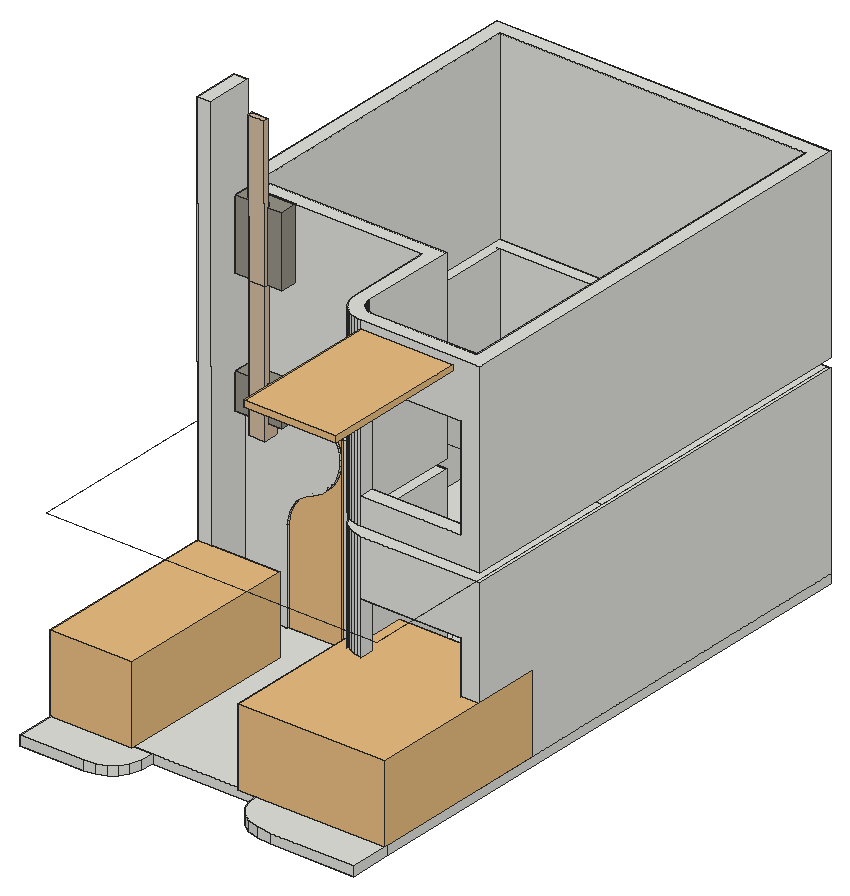
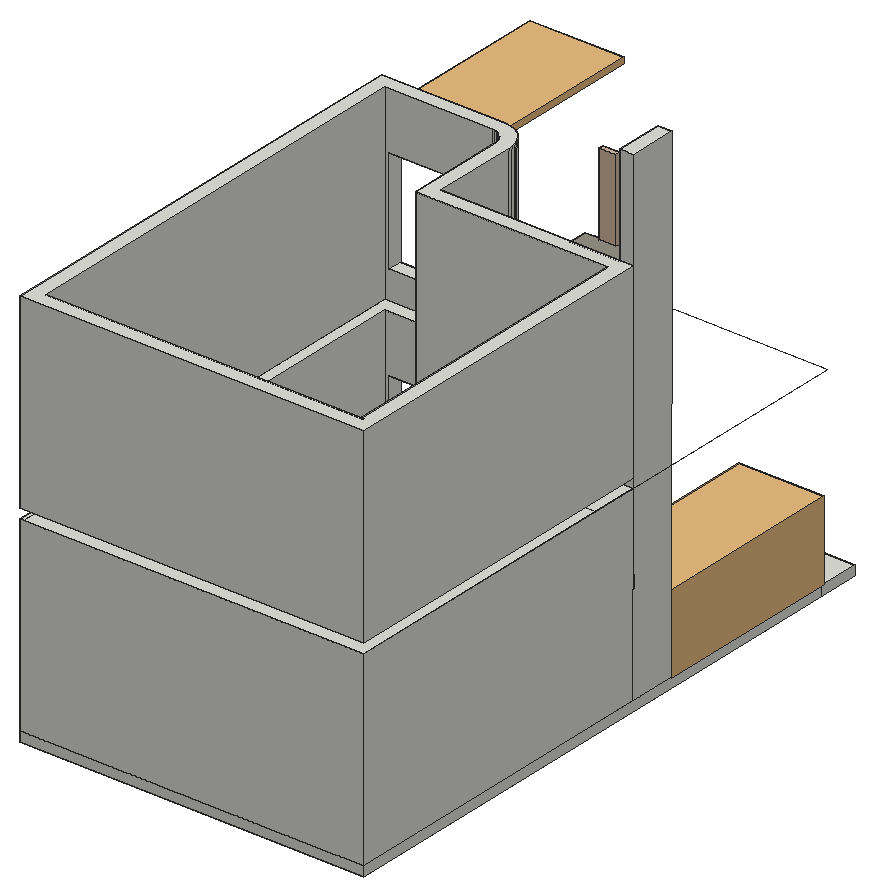
# SketchUp Ruby script. Lengths in inches.
U = 1.inch
M = Sketchup.active_model
def pt(a) = Geom::Point3d.new(a.map { |v| v * U })
def face(e, loops, mat)
  f = e.add_face(loops[0].map { |a| pt(a) })
  loops[1..].each { |l| e.add_face(l.map { |a| pt(a) }).erase! }
  f.material = f.back_material = mat if mat
  f
end
# faces: each face lists its corners as indices into pts; further lists are holes
def faces(e, pts, list, mat = nil) = list.each { |f| face(e, (f[0].is_a?(Array) ? f : [f]).map { |l| l.map { |i| pts[i] } }, mat) }
# xy, xz, yz: faces in a plane at the given z, y or x. An outline is a flat list of corners, or four numbers for a rectangle; further outlines are holes
def ring(l) = l.size == 4 ? [[l[0], l[1]], [l[2], l[1]], [l[2], l[3]], [l[0], l[3]]] : l.each_slice(2).to_a
def flat(e, list, mat, &to3) = list.each { |f| face(e, (f[0].is_a?(Array) ? f : [f]).map { |l| ring(l).map { |u, v| to3.(u, v) } }, mat) }
def xy(e, z, list, mat = nil) = flat(e, list, mat) { |x, y| [x, y, z] }
def xz(e, y, list, mat = nil) = flat(e, list, mat) { |x, z| [x, y, z] }
def yz(e, x, list, mat = nil) = flat(e, list, mat) { |y, z| [x, y, z] }
def lines(e, pts, list) = list.each { |a, b| e.add_line(pt(pts[a]), pt(pts[b])) }
# prism: a flat outline (further loops are holes) pulled along v
def prism(e, loops, v, mat = nil)
  f = face(e, loops, mat); d = Geom::Vector3d.new(v.map { |x| x * U })
  f.pushpull(f.normal.samedirection?(d) ? d.length : -d.length)
end
def box(e, o, s, mat = nil) = prism(e, [[o, [o[0] + s[0], o[1], o[2]], [o[0] + s[0], o[1] + s[1], o[2]], [o[0], o[1] + s[1], o[2]]]], [0, 0, s[2]], mat)
def at(x, y, z, deg = 0) = Geom::Transformation.translation(pt([x, y, z])) * Geom::Transformation.rotation(ORIGIN, Z_AXIS, deg.degrees)
def axes(o, x, y, z) = Geom::Transformation.new([*x, 0, *y, 0, *z, 0, *pt(o).to_a, 1])
def part(name) = M.definitions.add(name)
# library, detail: a bought-in or finely detailed component or shape, given as its bounding box
def library(name, o, s) = part(name).tap { |d| box(d.entities, o, s) }
def detail(e, o, s) = box(e.add_group.entities, o, s)
def put(e, d, t, mat = nil) = e.add_instance(d, t).tap { |i| i.material = mat if mat }
def group(e, t, mat = nil) = e.add_group.tap { |g| g.transformation = t; g.material = mat if mat }.entities
root = M.entities
M.materials.add("[Formica Graystone]").color = [149, 146, 135]
M.materials.add("[Formica Laminate Light]").color = [213, 189, 164]
M.materials.add("[Wood Cherry Original]").color = [152, 86, 42]
c1 = part("Group316\#3")
p = [[0,0,0],[0,0,-89.7],[-16.49,0,-89.7],[107.35,-183.05,0],[-107.35,-183.05,0],[107.35,183.05,0],
  [107.35,0,0],[-107.35,183.05,0],[16.49,0,-89.7],[-107.35,0,0],[0,0,-145.2]]
lines(c1.entities,p,[[0,1],[1,2],[3,4],[5,6],[7,5],[1,8],[9,0],[0,6],[8,10],[4,9],[6,3],[2,10],
  [9,7]])
c2 = part("Rectangle Light")
put(c2.entities,c1,at(0,0,0))
c3 = part("Group\#13")
prism(c3.entities,[[[0,0,0],[0,27,0],[84,27,0],[83.17,18.75,0],[80.68,12,0],[76.53,6.75,0],[70.71,3,0],[63.24,0.75,0],[54.1,0,0]]],[0,0,6])
c4 = library("Group\#11",[-9.29,0,0],[59.29,4,95])
c5 = library("Group\#10",[-0.5,-0.5,0],[35.9375,1,120.38])
c6 = library("Group123\#1",[-245.88,56.46,51.12],[36,6.2,84])
c7 = library("Group297\#3",[-33.91,-76.98,0],[95.34,119.86,50])
c8 = library("Group297\#2",[-33.91,-76.98,0],[95.34,119.86,50])
xy(root,48,[[132.2,27,195.57,32]])
xz(root,32,[[123.2,0,211.73,48]])
put(root,c2,axes([107.57,204.35,119.99],[1,0,0],[0,-1,0],[0,0,1]))
put(root,c3,axes([217.23,0,-6],[-1,0,0],[0,1,0],[0,0,1]))
g1 = group(root,at(29.625,105.98,-6))
xy(g1,0,[[-29.41,-78.98,-29.41,281.41,187.6,281.41,187.6,-78.98,178.93,-78.98,178.93,-75.77,174.22,-75.77,174.22,-78.98],[174.22,-78.98,174.22,-75.77,178.93,-75.77,178.93,-77.125,178.43,-77.82,177.68,-78.36,176.39,-78.79],[174.22,-78.98,176.39,-78.79,177.68,-78.36,178.43,-77.82,178.93,-77.125,178.93,-78.98]])
xy(g1,6,[[-29.41,-78.98,187.6,281.41]])
xz(g1,-78.98,[[-29.41,0,187.6,6]])
xz(g1,281.41,[[-29.41,0,187.6,6]])
yz(g1,-29.41,[[-78.98,0,281.41,6]])
yz(g1,187.6,[[-78.98,0,281.41,6]])
put(root,c3,axes([0.22,0,-6],[0.77,0,0],[0,1,0],[0,0,1]))
g2 = group(root,at(33.625,101.98,126))
xy(g2,0,[[106.8125,0,104.36,0.16,101.94,0.64,99.61,1.43,97.41,2.52,95.36,3.89,93.51,5.51,91.89,7.36,90.52,9.41,89.43,11.61,88.64,13.94,88.16,16.36,88,18.8125,88,72.51,40,72.51,40,81.51,97,81.51,97,18.8125,97.08,17.53,97.33,16.27,97.75,15.06,98.31,13.91,99.03,12.84,99.875,11.875,100.84,11.03,101.91,10.31,103.06,9.75,104.27,9.33,105.53,9.08,106.8125,9,174.6,9,174.6,276.41,0,276.41,0,285.41,183.6,285.41,183.6,0],[-33.41,72.51,-33.41,285.41,0,285.41,0,276.41,-24.41,276.41,-24.41,81.51,0,81.51,0,72.51],[0,72.51,40,81.51]])
xy(g2,18,[[106.8125,0,171.6,9]])
xy(g2,84,[[106.8125,0,171.6,9]])
xy(g2,120,[[[106.8125,0,183.6,0,183.6,285.41,-33.41,285.41,-33.41,72.51,88,72.51,88,18.8125,88.16,16.36,88.64,13.94,89.43,11.61,90.52,9.41,91.89,7.36,93.51,5.51,95.36,3.89,97.41,2.52,99.61,1.43,101.94,0.64,104.36,0.16],[106.8125,9,105.53,9.08,104.27,9.33,103.06,9.75,101.91,10.31,100.84,11.03,99.875,11.875,99.03,12.84,98.31,13.91,97.75,15.06,97.33,16.27,97.08,17.53,97,18.8125,97,81.51,-24.41,81.51,-24.41,276.41,174.6,276.41,174.6,9]]])
xz(g2,0,[[106.8125,0,183.6,0,183.6,120,106.8125,120,106.8125,84,171.6,84,171.6,18,106.8125,18]])
xz(g2,9,[[106.8125,0,106.8125,18,171.6,18,171.6,84,106.8125,84,106.8125,120,174.6,120,174.6,0]])
xz(g2,72.51,[[-33.41,0,88,120]])
xz(g2,81.51,[[-24.41,0,97,120]])
xz(g2,276.41,[[-26.08,0,-24.41,120],[-24.41,0,174.6,120]])
xz(g2,285.41,[[-33.41,0,183.6,120]])
yz(g2,-33.41,[[42.875,-126.09,41.97,182.5,71.97,182.58,72.51,0,72.875,-126],[72.51,0,285.41,120]])
yz(g2,-24.41,[[42.875,-126.09,72.875,-126,72.51,0,71.97,182.58,41.97,182.5],[81.51,0,276.41,120]])
yz(g2,88,[[18.8125,0,72.51,120]])
yz(g2,97,[[18.8125,0,81.51,120]])
yz(g2,106.8125,[[0,18,9,84]])
yz(g2,171.6,[[0,18,9,84]])
yz(g2,174.6,[[9,0,276.41,120]])
yz(g2,183.6,[[0,0,285.41,120]])
p = [[-24.41,41.97,182.5],[-33.41,41.97,182.5],[-33.41,42.875,-126.09],[-24.41,42.875,-126.09],[-33.41,72.875,-126],[-24.41,72.875,-126],
  [-33.41,72.51,0],[-24.41,72.51,0],[104.36,0.16,0],[106.8125,0,0],[106.8125,0,18],[106.8125,0,84],
  [106.8125,0,120],[104.36,0.16,120],[101.94,0.64,0],[101.94,0.64,120],[99.61,1.43,0],[99.61,1.43,120],
  [97.41,2.52,0],[97.41,2.52,120],[95.36,3.89,0],[95.36,3.89,120],[93.51,5.51,0],[93.51,5.51,120],
  [91.89,7.36,0],[91.89,7.36,120],[90.52,9.41,0],[90.52,9.41,120],[106.8125,9,0],[105.53,9.08,0],
  [105.53,9.08,120],[106.8125,9,120],[106.8125,9,84],[106.8125,9,18],[104.27,9.33,0],[104.27,9.33,120],
  [103.06,9.75,0],[103.06,9.75,120],[89.43,11.61,0],[89.43,11.61,120],[101.91,10.31,0],[101.91,10.31,120],
  [100.84,11.03,0],[100.84,11.03,120],[99.875,11.875,0],[99.875,11.875,120],[88.64,13.94,0],[88.64,13.94,120],
  [99.03,12.84,0],[99.03,12.84,120],[98.31,13.91,0],[98.31,13.91,120],[88.16,16.36,0],[88.16,16.36,120],
  [97.75,15.06,0],[97.75,15.06,120],[97.33,16.27,0],[97.33,16.27,120],[97.08,17.53,0],[97.08,17.53,120],
  [88,18.8125,0],[88,18.8125,120],[97,18.8125,0],[97,18.8125,120],[-33.41,71.97,182.58],[-24.41,71.97,182.58]]
faces(g2,p,[[0,1,2,3],[4,5,3,2],[6,7,5,4],[8,9,10,11,12,13],[14,8,13,15],[16,14,15,17],[18,16,17,19],[20,18,19,21],
  [22,20,21,23],[24,22,23,25],[26,24,25,27],[28,29,30,31,32,33],[29,34,35,30],[34,36,37,35],[38,26,27,39],[36,40,41,37],
  [40,42,43,41],[42,44,45,43],[46,38,39,47],[44,48,49,45],[48,50,51,49],[52,46,47,53],[50,54,55,51],[54,56,57,55],
  [56,58,59,57],[60,52,53,61],[58,62,63,59],[64,65,7,6],[1,0,65,64]])
g3 = group(g2,at(-24.41,72.34,57.67),"[Formica Graystone]")
prism(g3,[[[0,0.18,-63.22],[30.33,0.35,-63.22],[30.39,-10.65,-63.25],[0.0625,-10.81,-63.25]]],[0,-0.07,23.04])
p = [[0.0625,-11.18,62.3],[-0.01,0.82,62.33],[-0.01,0.95,17.01],[0,-0.05,17],[0.0625,-11.05,16.97],[10.46,-10.99,16.97],
  [10.46,-11.125,62.3],[30.39,-11.01,62.3],[20.9375,-11.07,62.3],[20.9375,-10.93,16.97],[30.39,-10.88,16.97],[30.32,1.12,17.01],
  [30.32,0.99,62.33],[0,0.12,-40.18]]
faces(g3,p,[[0,1,2,3,4],[4,5,6,0],[7,8,9,10],[10,9,5,4,3,2,11],[10,11,12,7],[12,11,2,1],[7,12,1,0,6,8]])
lines(g3,p,[[3,13]])
g4 = group(g3,at(10.46,-10.93,16.97),"[Formica Laminate Light]")
p = [[-0.01,0.94,0],[-0.01,1.18,-80.22],[-0.06,11.03,-80.1875],[-0.06,11.0625,-90.1875],[0.01,-1.79,-90.23],[0.01,-2.06,-0.01],
  [10.49,-1.74,-90.23],[10.49,-2,-0.01],[10.42,11.12,-90.1875],[10.42,11.09,-80.1875],[10.48,1.23,-80.22],[10.48,1,0],
  [10.49,-2.28,96.77],[0.01,-2.34,96.77],[-0.01,0.66,96.78],[10.48,0.72,96.78]]
faces(g4,p,[[0,1,2,3,4,5],[5,4,6,7],[7,6,8,9,10,11],[8,6,4,3],[3,2,9,8],[11,10,1,0],[1,10,9,2],[12,13,5,7],
  [13,14,0,5],[15,12,7,11],[5,7,11,0],[14,15,11,0],[14,13,12,15]])
put(g2,c4,axes([116.1,0,111.06],[1,0,0],[0,0,1],[0,-1,0]))
g5 = group(root,at(33.625,101.98,0))
xy(g5,0,[[106.8125,0,104.36,0.16,101.94,0.64,99.61,1.43,97.41,2.52,95.36,3.89,93.51,5.51,91.89,7.36,90.52,9.41,89.43,11.61,88.64,13.94,88.16,16.36,88,18.8125,88,72.51,76,72.51,76,81.51,97,81.51,97,18.8125,97.08,17.53,97.33,16.27,97.75,15.06,98.31,13.91,99.03,12.84,99.875,11.875,100.84,11.03,101.91,10.31,103.06,9.75,104.27,9.33,105.53,9.08,106.8125,9,174.6,9,174.6,276.41,0,276.41,0,285.41,183.6,285.41,183.6,0],[-33.41,69.51,-33.41,285.41,0,285.41,0,276.41,-24.41,276.41,-24.41,81.51,0,81.51,0,69.51],[0,69.51,0,81.51,40,81.51,40,72.51,2.51,72.51,2.51,69.51],[2.51,69.51,3.51,71.01]])
xy(g5,18,[[106.8125,0,171.6,9]])
xy(g5,84,[[106.8125,0,171.6,9],[40,72.51,76,81.51]])
xy(g5,120,[[[106.8125,0,183.6,0,183.6,285.41,-33.41,285.41,-33.41,69.51,33.73,69.51,33.73,72.51,88,72.51,88,18.8125,88.16,16.36,88.64,13.94,89.43,11.61,90.52,9.41,91.89,7.36,93.51,5.51,95.36,3.89,97.41,2.52,99.61,1.43,101.94,0.64,104.36,0.16],[106.8125,9,105.53,9.08,104.27,9.33,103.06,9.75,101.91,10.31,100.84,11.03,99.875,11.875,99.03,12.84,98.31,13.91,97.75,15.06,97.33,16.27,97.08,17.53,97,18.8125,97,81.51,-24.41,81.51,-24.41,276.41,174.6,276.41,174.6,9]]])
xz(g5,0,[[106.8125,0,183.6,0,183.6,120,106.8125,120,106.8125,84,171.6,84,171.6,18,106.8125,18]])
xz(g5,9,[[106.8125,0,106.8125,18,171.6,18,171.6,84,106.8125,84,106.8125,120,174.6,120,174.6,0]])
xz(g5,69.51,[[-33.41,0,3.51,0,3.51,59.97,3.64,62.47,4.01,64.91,4.64,67.3,5.5,69.62,6.6,71.83,7.91,73.92,9.43,75.87,11.14,77.65,13.03,79.25,15.07,80.65,17.24,81.83,19.57,82.81,23,84.33,26.24,86.35,29.16,88.8,31.72,91.63,33.84,94.8,35.51,98.23,36.68,101.86,37.33,105.62,37.44,109.43,37.03,113.22,36.08,116.92,34.66,120.38,33.73,120,-33.41,120]])
xz(g5,72.51,[[2.51,0,40,0,40,84,76,84,76,0,88,0,88,120,33.73,120,35.13,116.6,36.04,113.04,36.44,109.39,36.33,105.72,35.71,102.1,34.58,98.6,32.98,95.3,30.92,92.25,28.47,89.52,25.65,87.16,22.53,85.22,19.17,83.73,16.8,82.74,14.54,81.5,12.42,80.05,10.46,78.38,8.68,76.53,7.09,74.5,5.72,72.32,4.58,70.01,3.68,67.6,3.03,65.11,2.64,62.57,2.51,60]])
xz(g5,81.51,[[-24.41,0,-24.41,120,97,120,97,0,76,0,76,84,40,84,40,0]])
xz(g5,276.41,[[-26.08,0,-24.41,120],[-24.41,0,174.6,120]])
xz(g5,285.41,[[-33.41,0,183.6,120]])
yz(g5,-33.41,[[69.51,0,285.41,120]])
yz(g5,-24.41,[[81.51,0,276.41,120]])
yz(g5,2.51,[[71.01,0,72.51,60]])
yz(g5,3.51,[[69.51,0,71.01,59.97]])
yz(g5,40,[[72.51,0,81.51,84]])
yz(g5,76,[[72.51,0,81.51,84]])
yz(g5,88,[[18.8125,0,72.51,120]])
yz(g5,97,[[18.8125,0,81.51,120]])
yz(g5,106.8125,[[0,18,9,84]])
yz(g5,171.6,[[0,18,9,84]])
yz(g5,174.6,[[9,0,276.41,120]])
yz(g5,183.6,[[0,0,285.41,120]])
p = [[104.36,0.16,0],[106.8125,0,0],[106.8125,0,18],[106.8125,0,84],[106.8125,0,120],[104.36,0.16,120],
  [101.94,0.64,0],[101.94,0.64,120],[99.61,1.43,0],[99.61,1.43,120],[97.41,2.52,0],[97.41,2.52,120],
  [95.36,3.89,0],[95.36,3.89,120],[93.51,5.51,0],[93.51,5.51,120],[91.89,7.36,0],[91.89,7.36,120],
  [90.52,9.41,0],[90.52,9.41,120],[106.8125,9,0],[105.53,9.08,0],[105.53,9.08,120],[106.8125,9,120],
  [106.8125,9,84],[106.8125,9,18],[104.27,9.33,0],[104.27,9.33,120],[103.06,9.75,0],[103.06,9.75,120],
  [89.43,11.61,0],[89.43,11.61,120],[101.91,10.31,0],[101.91,10.31,120],[100.84,11.03,0],[100.84,11.03,120],
  [99.875,11.875,0],[99.875,11.875,120],[88.64,13.94,0],[88.64,13.94,120],[99.03,12.84,0],[99.03,12.84,120],
  [98.31,13.91,0],[98.31,13.91,120],[88.16,16.36,0],[88.16,16.36,120],[97.75,15.06,0],[97.75,15.06,120],
  [97.33,16.27,0],[97.33,16.27,120],[97.08,17.53,0],[97.08,17.53,120],[88,18.8125,0],[88,18.8125,120],
  [97,18.8125,0],[97,18.8125,120],[3.51,69.51,59.97],[3.51,71.01,59.97],[3.64,71.01,62.47],[3.64,69.51,62.47],
  [2.64,72.51,62.57],[2.64,71.01,62.57],[2.51,71.01,60],[2.51,72.51,60],[4.01,71.01,64.91],[4.01,69.51,64.91],
  [3.03,72.51,65.11],[3.03,71.01,65.11],[4.64,71.01,67.3],[4.64,69.51,67.3],[3.68,72.51,67.6],[3.68,71.01,67.6],
  [5.5,71.01,69.62],[5.5,69.51,69.62],[4.58,72.51,70.01],[4.58,71.01,70.01],[6.6,71.01,71.83],[6.6,69.51,71.83],
  [5.72,72.51,72.32],[5.72,71.01,72.32],[7.91,71.01,73.92],[7.91,69.51,73.92],[7.09,72.51,74.5],[7.09,71.01,74.5],
  [9.43,71.01,75.87],[9.43,69.51,75.87],[8.68,72.51,76.53],[8.68,71.01,76.53],[11.14,69.51,77.65],[11.14,71.01,77.65],
  [10.46,72.51,78.38],[10.46,71.01,78.38],[13.03,71.01,79.25],[13.03,69.51,79.25],[12.42,72.51,80.05],[12.42,71.01,80.05],
  [15.07,71.01,80.65],[15.07,69.51,80.65],[14.54,72.51,81.5],[14.54,71.01,81.5],[17.24,71.01,81.83],[17.24,69.51,81.83],
  [16.8,72.51,82.74],[16.8,71.01,82.74],[19.57,71.01,82.81],[19.57,69.51,82.81],[19.17,72.51,83.73],[19.17,71.01,83.73],
  [23,71.01,84.33],[23,69.51,84.33],[22.53,72.51,85.22],[22.53,71.01,85.22],[26.24,71.01,86.35],[26.24,69.51,86.35],
  [25.65,72.51,87.16],[25.65,71.01,87.16],[29.16,71.01,88.8],[29.16,69.51,88.8],[28.47,72.51,89.52],[28.47,71.01,89.52],
  [31.72,69.51,91.63],[31.72,71.01,91.63],[30.92,72.51,92.25],[30.92,71.01,92.25],[33.84,69.51,94.8],[33.84,71.01,94.8],
  [32.98,72.51,95.3],[32.98,71.01,95.3],[35.51,71.01,98.23],[35.51,69.51,98.23],[34.58,72.51,98.6],[34.58,71.01,98.6],
  [36.68,71.01,101.86],[36.68,69.51,101.86],[35.71,72.51,102.1],[35.71,71.01,102.1],[37.33,71.01,105.62],[37.33,69.51,105.62],
  [36.33,72.51,105.72],[36.33,71.01,105.72],[37.44,71.01,109.43],[37.44,69.51,109.43],[36.44,72.51,109.39],[36.44,71.01,109.39],
  [37.03,71.01,113.22],[37.03,69.51,113.22],[36.04,72.51,113.04],[36.04,71.01,113.04],[35.13,72.51,116.6],[35.13,71.01,116.6],
  [36.08,71.01,116.92],[36.08,69.51,116.92],[33.73,72.51,120],[33.73,71.01,120],[34.66,71.01,120.38],[34.66,69.51,120.38],
  [33.73,69.51,120],[2.51,69.51,60],[19.17,69.51,83.73]]
faces(g5,p,[[0,1,2,3,4,5],[6,0,5,7],[8,6,7,9],[10,8,9,11],[12,10,11,13],[14,12,13,15],[16,14,15,17],[18,16,17,19],
  [20,21,22,23,24,25],[21,26,27,22],[26,28,29,27],[30,18,19,31],[28,32,33,29],[32,34,35,33],[34,36,37,35],[38,30,31,39],
  [36,40,41,37],[40,42,43,41],[44,38,39,45],[42,46,47,43],[46,48,49,47],[48,50,51,49],[52,44,45,53],[50,54,55,51],
  [56,57,58,59],[60,61,62,63],[59,58,64,65],[66,67,61,60],[65,64,68,69],[70,71,67,66],[69,68,72,73],[74,75,71,70],
  [73,72,76,77],[78,79,75,74],[77,76,80,81],[82,83,79,78],[81,80,84,85],[86,87,83,82],[88,85,84,89],[90,91,87,86],
  [88,89,92,93],[94,95,91,90],[93,92,96,97],[98,99,95,94],[97,96,100,101],[102,103,99,98],[101,100,104,105],[106,107,103,102],
  [105,104,108,109],[110,111,107,106],[109,108,112,113],[114,115,111,110],[113,112,116,117],[118,119,115,114],[120,117,116,121],[122,123,119,118],
  [124,120,121,125],[126,127,123,122],[124,125,128,129],[130,131,127,126],[129,128,132,133],[134,135,131,130],[133,132,136,137],[138,139,135,134],
  [137,136,140,141],[142,143,139,138],[141,140,144,145],[146,147,143,142],[148,149,147,146],[145,144,150,151],[152,153,149,148],[151,150,154,155],
  [156,155,154,153]])
lines(g5,p,[[62,157],[107,158]])
put(g5,c5,at(2.51,71.01,0))
put(root,c6,axes([-136.25,118.03,-51.12],[-1,0,0],[0,1,0],[0,0,1]),"[Wood Cherry Original]")
put(root,c7,axes([18.71,101.98,0],[0.56,0,0],[0,1,0],[0,0,1]))
put(root,c8,axes([183.32,101.98,0],[-1,0,0],[0,1,0],[0,0,1]))
